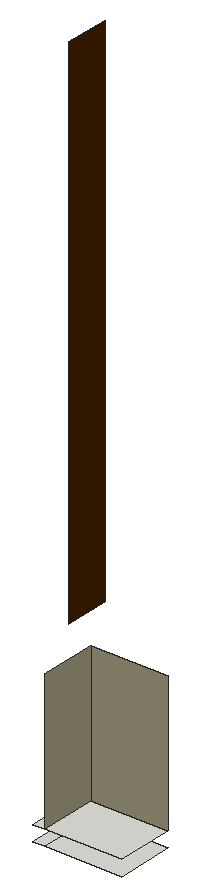
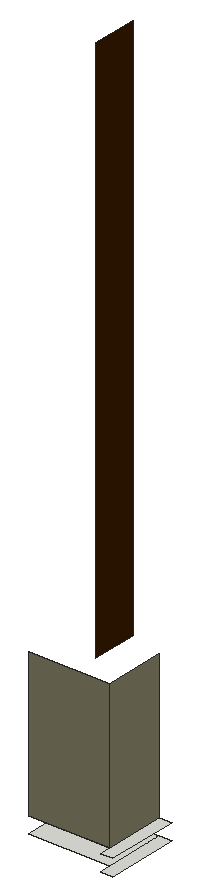
# SketchUp Ruby script. Lengths in inches.
U = 1.inch
M = Sketchup.active_model
def pt(a) = Geom::Point3d.new(a.map { |v| v * U })
def face(e, loops, mat)
  f = e.add_face(loops[0].map { |a| pt(a) })
  loops[1..].each { |l| e.add_face(l.map { |a| pt(a) }).erase! }
  f.material = f.back_material = mat if mat
  f
end
# faces: each face lists its corners as indices into pts; further lists are holes
def faces(e, pts, list, mat = nil) = list.each { |f| face(e, (f[0].is_a?(Array) ? f : [f]).map { |l| l.map { |i| pts[i] } }, mat) }
# xy, xz, yz: faces in a plane at the given z, y or x. An outline is a flat list of corners, or four numbers for a rectangle; further outlines are holes
def ring(l) = l.size == 4 ? [[l[0], l[1]], [l[2], l[1]], [l[2], l[3]], [l[0], l[3]]] : l.each_slice(2).to_a
def flat(e, list, mat, &to3) = list.each { |f| face(e, (f[0].is_a?(Array) ? f : [f]).map { |l| ring(l).map { |u, v| to3.(u, v) } }, mat) }
def xy(e, z, list, mat = nil) = flat(e, list, mat) { |x, y| [x, y, z] }
def xz(e, y, list, mat = nil) = flat(e, list, mat) { |x, z| [x, y, z] }
def yz(e, x, list, mat = nil) = flat(e, list, mat) { |y, z| [x, y, z] }
def lines(e, pts, list) = list.each { |a, b| e.add_line(pt(pts[a]), pt(pts[b])) }
# prism: a flat outline (further loops are holes) pulled along v
def prism(e, loops, v, mat = nil)
  f = face(e, loops, mat); d = Geom::Vector3d.new(v.map { |x| x * U })
  f.pushpull(f.normal.samedirection?(d) ? d.length : -d.length)
end
def box(e, o, s, mat = nil) = prism(e, [[o, [o[0] + s[0], o[1], o[2]], [o[0] + s[0], o[1] + s[1], o[2]], [o[0], o[1] + s[1], o[2]]]], [0, 0, s[2]], mat)
def at(x, y, z, deg = 0) = Geom::Transformation.translation(pt([x, y, z])) * Geom::Transformation.rotation(ORIGIN, Z_AXIS, deg.degrees)
def axes(o, x, y, z) = Geom::Transformation.new([*x, 0, *y, 0, *z, 0, *pt(o).to_a, 1])
def part(name) = M.definitions.add(name)
# library, detail: a bought-in or finely detailed component or shape, given as its bounding box
def library(name, o, s) = part(name).tap { |d| box(d.entities, o, s) }
def detail(e, o, s) = box(e.add_group.entities, o, s)
def put(e, d, t, mat = nil) = e.add_instance(d, t).tap { |i| i.material = mat if mat }
def group(e, t, mat = nil) = e.add_group.tap { |g| g.transformation = t; g.material = mat if mat }.entities
root = M.entities
M.materials.add("[Color C08]").color = [63, 31, 0]
M.materials.add("[Stone Coursed Rough]").color = [155, 150, 122]
xy(root,95.36,[[165.87,203.17,168.55,219.06],[168.55,203.17,186.24,216.5]])
xy(root,98.875,[[165.87,203.17,168.55,219.06],[168.55,203.17,186.24,216.5]])
xz(root,216.5,[[168.55,98.875,186.24,130.875]],"[Stone Coursed Rough]")
yz(root,168.19,[[210.73,137.875,220.88,257.875]],"[Color C08]")
yz(root,168.55,[[203.17,98.875,216.5,130.875]],"[Stone Coursed Rough]")
